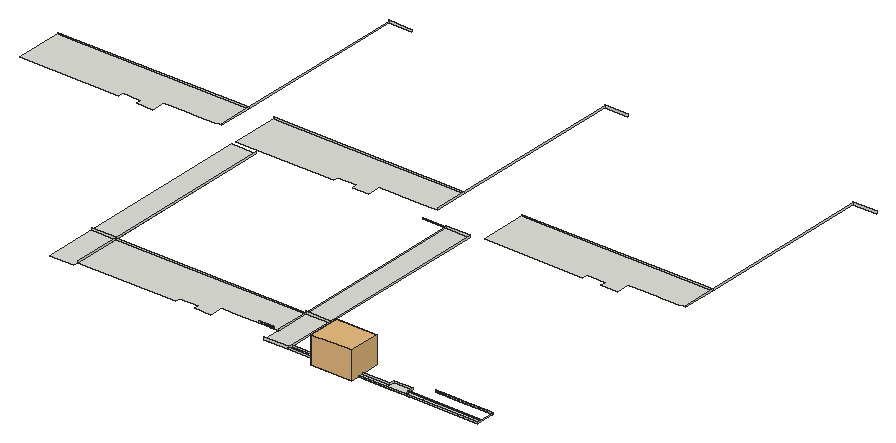
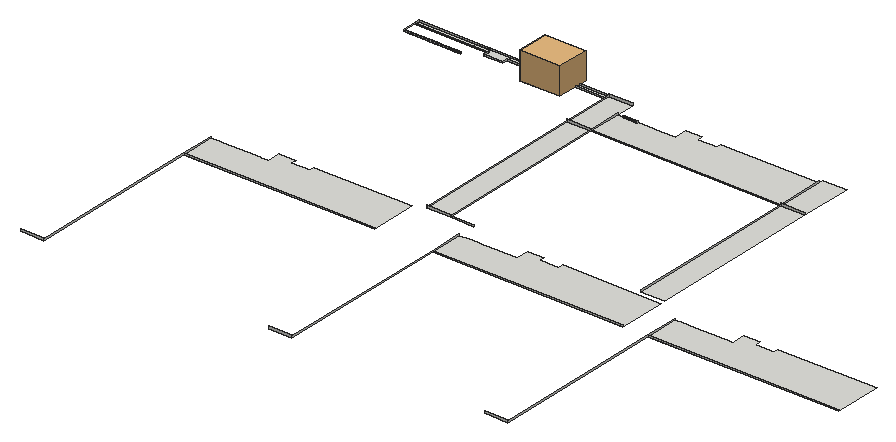
# SketchUp Ruby script. Lengths in inches.
U = 1.inch
M = Sketchup.active_model
def pt(a) = Geom::Point3d.new(a.map { |v| v * U })
def face(e, loops, mat)
  f = e.add_face(loops[0].map { |a| pt(a) })
  loops[1..].each { |l| e.add_face(l.map { |a| pt(a) }).erase! }
  f.material = f.back_material = mat if mat
  f
end
# faces: each face lists its corners as indices into pts; further lists are holes
def faces(e, pts, list, mat = nil) = list.each { |f| face(e, (f[0].is_a?(Array) ? f : [f]).map { |l| l.map { |i| pts[i] } }, mat) }
# xy, xz, yz: faces in a plane at the given z, y or x. An outline is a flat list of corners, or four numbers for a rectangle; further outlines are holes
def ring(l) = l.size == 4 ? [[l[0], l[1]], [l[2], l[1]], [l[2], l[3]], [l[0], l[3]]] : l.each_slice(2).to_a
def flat(e, list, mat, &to3) = list.each { |f| face(e, (f[0].is_a?(Array) ? f : [f]).map { |l| ring(l).map { |u, v| to3.(u, v) } }, mat) }
def xy(e, z, list, mat = nil) = flat(e, list, mat) { |x, y| [x, y, z] }
def xz(e, y, list, mat = nil) = flat(e, list, mat) { |x, z| [x, y, z] }
def yz(e, x, list, mat = nil) = flat(e, list, mat) { |y, z| [x, y, z] }
def lines(e, pts, list) = list.each { |a, b| e.add_line(pt(pts[a]), pt(pts[b])) }
# prism: a flat outline (further loops are holes) pulled along v
def prism(e, loops, v, mat = nil)
  f = face(e, loops, mat); d = Geom::Vector3d.new(v.map { |x| x * U })
  f.pushpull(f.normal.samedirection?(d) ? d.length : -d.length)
end
def box(e, o, s, mat = nil) = prism(e, [[o, [o[0] + s[0], o[1], o[2]], [o[0] + s[0], o[1] + s[1], o[2]], [o[0], o[1] + s[1], o[2]]]], [0, 0, s[2]], mat)
def at(x, y, z, deg = 0) = Geom::Transformation.translation(pt([x, y, z])) * Geom::Transformation.rotation(ORIGIN, Z_AXIS, deg.degrees)
def axes(o, x, y, z) = Geom::Transformation.new([*x, 0, *y, 0, *z, 0, *pt(o).to_a, 1])
def part(name) = M.definitions.add(name)
# library, detail: a bought-in or finely detailed component or shape, given as its bounding box
def library(name, o, s) = part(name).tap { |d| box(d.entities, o, s) }
def detail(e, o, s) = box(e.add_group.entities, o, s)
def put(e, d, t, mat = nil) = e.add_instance(d, t).tap { |i| i.material = mat if mat }
def group(e, t, mat = nil) = e.add_group.tap { |g| g.transformation = t; g.material = mat if mat }.entities
root = M.entities
c1 = library("Sem+nome (1)",[20.77,3.52,-2.22],[96.42,122.82,82.56])
xy(root,-12.3125,[[1063.02,147.25,1134.71,305.58],[1713.52,147.25,1785.21,305.58],[1785.21,147.25,1886.4,162.52],[1950.69,147.25,1952.69,147.38,1954.64,147.77,1956.53,148.41,1958.33,149.3,1959.99,150.4,1961.49,151.72,1962.8,153.22,1963.91,154.88,1964.8,156.67,1965.4375,158.57,1965.83,160.52,1965.96,162.52,2083.4,162.52,2083.4,147.25],[2083.4,147.25,2083.4,178.0625,2140.42,178.0625,2140.42,162.33,2140.55,160.36,2140.93,158.43,2141.57,156.56,2142.4375,154.79,2143.53,153.15,2144.84,151.67,2146.32,150.37,2147.96,149.27,2149.73,148.4,2151.6,147.76,2153.53,147.38,2155.5,147.25],
  [2155.5,147.25,2153.53,147.38,2151.6,147.76,2149.73,148.4,2147.96,149.27,2146.32,150.37,2144.84,151.67,2143.53,153.15,2142.4375,154.79,2141.57,156.56,2140.93,158.43,2140.55,160.36,2140.42,162.33,2189.5,162.33,2189.5,147.25],[2189.5,147.25,2364.02,162.33],[1489.92,162.33,1489.92,178.0625,1432.9,178.0625,1432.9,162.52,1134.71,162.52,1134.71,305.58,1713.52,305.58,1713.52,203.875,1697.375,203.875,1697.375,204.875,1696.625,204.875,1696.625,203.875,1693.375,203.875,1693.375,204.875,1692.625,204.875,1692.625,203.875,1689.375,203.875,1689.375,204.875,1688.625,204.875,1688.625,203.875,1685.375,203.875,1685.375,204.875,1684.625,204.875,1684.625,203.875,1681.375,203.875,1681.375,204.875,1680.625,204.875,1680.625,203.875,1677.375,203.875,1677.375,204.875,1676.625,204.875,1676.625,203.875,1673.375,203.875,1673.375,204.875,1672.625,204.875,1672.625,203.875,1669.375,203.875,1669.375,204.875,1668.625,204.875,1668.625,203.875,1665.375,203.875,1665.375,204.875,1664.625,204.875,1664.625,203.875,1661.375,203.875,1661.375,204.875,1660.625,204.875,1660.625,203.875,1657.375,203.875,1657.375,204.875,1656.625,204.875,1656.625,203.875,1653.375,203.875,1653.375,204.875,1652.625,204.875,1652.625,203.875,1649.375,203.875,1649.375,204.875,1648.625,204.875,1648.625,203.875,1645.375,203.875,1645.375,204.875,1644.625,204.875,1644.625,203.875,1641.375,203.875,1641.375,204.875,1640.625,204.875,1640.625,203.875,1637.375,203.875,1637.375,204.875,1636.625,204.875,1636.625,203.875,1633.375,203.875,1633.375,204.875,1632.625,204.875,1632.625,203.875,1629.375,203.875,1629.375,204.875,1628.625,204.875,1628.625,203.875,1625.375,203.875,1625.375,204.875,1624.625,204.875,1624.625,203.875,1621.375,203.875,1621.375,204.875,1620.625,204.875,1620.625,203.875,1617.375,203.875,1617.375,204.875,1616.625,204.875,1616.625,203.875,1613.375,203.875,1613.375,204.875,1612.625,204.875,1612.625,203.875,1609.375,203.875,1609.375,204.875,1608.625,204.875,1608.625,203.875,1605.375,203.875,1605.375,204.875,1604.625,204.875,1604.625,203.875,1601.375,203.875,1601.375,204.875,1600.625,204.875,1600.625,203.875,1597.375,203.875,1597.375,204.875,1596.625,204.875,1596.625,203.875,1593.375,203.875,1593.375,204.875,1592.625,204.875,1592.625,203.875,1589.375,203.875,1589.375,204.875,1588.625,204.875,1588.625,203.875,1585.375,203.875,1585.375,204.875,1584.625,204.875,1584.625,203.875,1581.375,203.875,1581.375,204.875,1580.625,204.875,1580.625,203.875,1577.375,203.875,1577.375,204.875,1576.625,204.875,1576.625,203.875,1573.375,203.875,1573.375,204.875,1572.625,204.875,1572.625,203.875,1569.375,203.875,1569.375,204.875,1568.625,204.875,1568.625,203.875,1565.375,203.875,1565.375,204.875,1564.625,204.875,1564.625,203.875,1561.375,203.875,1561.375,204.875,1560.625,204.875,1560.625,203.875,1557.375,203.875,1557.375,204.875,1556.625,204.875,1556.625,203.875,1553.375,203.875,1553.375,204.875,1552.625,204.875,1552.625,203.875,1549.375,203.875,1549.375,204.875,1548.625,204.875,1548.625,203.875,1545.375,203.875,1545.375,204.875,1544.625,204.875,1544.625,203.875,1541.375,203.875,1541.375,204.875,1540.625,204.875,1540.625,203.875,1539,203.875,1539,162.33],[1063.02,305.58,1134.71,838.14],[1713.52,305.58,1785.21,838.14],
  [762.73,853.22,762.73,868.96,705.71,868.96,705.71,853.41,407.52,853.41,407.52,996.48,986.33,996.48,986.33,894.77,970.1875,894.77,970.1875,895.77,969.4375,895.77,969.4375,894.77,966.1875,894.77,966.1875,895.77,965.4375,895.77,965.4375,894.77,962.1875,894.77,962.1875,895.77,961.4375,895.77,961.4375,894.77,958.1875,894.77,958.1875,895.77,957.4375,895.77,957.4375,894.77,954.1875,894.77,954.1875,895.77,953.4375,895.77,953.4375,894.77,950.1875,894.77,950.1875,895.77,949.4375,895.77,949.4375,894.77,946.1875,894.77,946.1875,895.77,945.4375,895.77,945.4375,894.77,942.1875,894.77,942.1875,895.77,941.4375,895.77,941.4375,894.77,938.1875,894.77,938.1875,895.77,937.4375,895.77,937.4375,894.77,934.1875,894.77,934.1875,895.77,933.4375,895.77,933.4375,894.77,930.1875,894.77,930.1875,895.77,929.4375,895.77,929.4375,894.77,926.1875,894.77,926.1875,895.77,925.4375,895.77,925.4375,894.77,922.1875,894.77,922.1875,895.77,921.4375,895.77,921.4375,894.77,918.1875,894.77,918.1875,895.77,917.4375,895.77,917.4375,894.77,914.1875,894.77,914.1875,895.77,913.4375,895.77,913.4375,894.77,910.1875,894.77,910.1875,895.77,909.4375,895.77,909.4375,894.77,906.1875,894.77,906.1875,895.77,905.4375,895.77,905.4375,894.77,902.1875,894.77,902.1875,895.77,901.4375,895.77,901.4375,894.77,898.1875,894.77,898.1875,895.77,897.4375,895.77,897.4375,894.77,894.1875,894.77,894.1875,895.77,893.4375,895.77,893.4375,894.77,890.1875,894.77,890.1875,895.77,889.4375,895.77,889.4375,894.77,886.1875,894.77,886.1875,895.77,885.4375,895.77,885.4375,894.77,882.1875,894.77,882.1875,895.77,881.4375,895.77,881.4375,894.77,878.1875,894.77,878.1875,895.77,877.4375,895.77,877.4375,894.77,874.1875,894.77,874.1875,895.77,873.4375,895.77,873.4375,894.77,870.1875,894.77,870.1875,895.77,869.4375,895.77,869.4375,894.77,866.1875,894.77,866.1875,895.77,865.4375,895.77,865.4375,894.77,862.1875,894.77,862.1875,895.77,861.4375,895.77,861.4375,894.77,858.1875,894.77,858.1875,895.77,857.4375,895.77,857.4375,894.77,854.1875,894.77,854.1875,895.77,853.4375,895.77,853.4375,894.77,850.1875,894.77,850.1875,895.77,849.4375,895.77,849.4375,894.77,846.1875,894.77,846.1875,895.77,845.4375,895.77,845.4375,894.77,842.1875,894.77,842.1875,895.77,841.4375,895.77,841.4375,894.77,838.1875,894.77,838.1875,895.77,837.4375,895.77,837.4375,894.77,834.1875,894.77,834.1875,895.77,833.4375,895.77,833.4375,894.77,830.1875,894.77,830.1875,895.77,829.4375,895.77,829.4375,894.77,826.1875,894.77,826.1875,895.77,825.4375,895.77,825.4375,894.77,822.1875,894.77,822.1875,895.77,821.4375,895.77,821.4375,894.77,818.1875,894.77,818.1875,895.77,817.4375,895.77,817.4375,894.77,814.1875,894.77,814.1875,895.77,813.4375,895.77,813.4375,894.77,811.8125,894.77,811.8125,853.22],[1418.23,853.22,1418.23,868.96,1361.21,868.96,1361.21,853.41,1063.02,853.41,1063.02,996.48,1641.83,996.48,1641.83,894.77,1625.6875,894.77,1625.6875,895.77,1624.9375,895.77,1624.9375,894.77,1621.6875,894.77,1621.6875,895.77,1620.9375,895.77,1620.9375,894.77,1617.6875,894.77,1617.6875,895.77,1616.9375,895.77,1616.9375,894.77,1613.6875,894.77,1613.6875,895.77,1612.9375,895.77,1612.9375,894.77,1609.6875,894.77,1609.6875,895.77,1608.9375,895.77,1608.9375,894.77,1605.6875,894.77,1605.6875,895.77,1604.9375,895.77,1604.9375,894.77,1601.6875,894.77,1601.6875,895.77,1600.9375,895.77,1600.9375,894.77,1597.6875,894.77,1597.6875,895.77,1596.9375,895.77,1596.9375,894.77,1593.6875,894.77,1593.6875,895.77,1592.9375,895.77,1592.9375,894.77,1589.6875,894.77,1589.6875,895.77,1588.9375,895.77,1588.9375,894.77,1585.6875,894.77,1585.6875,895.77,1584.9375,895.77,1584.9375,894.77,1581.6875,894.77,1581.6875,895.77,1580.9375,895.77,1580.9375,894.77,1577.6875,894.77,1577.6875,895.77,1576.9375,895.77,1576.9375,894.77,1573.6875,894.77,1573.6875,895.77,1572.9375,895.77,1572.9375,894.77,1569.6875,894.77,1569.6875,895.77,1568.9375,895.77,1568.9375,894.77,1565.6875,894.77,1565.6875,895.77,1564.9375,895.77,1564.9375,894.77,1561.6875,894.77,1561.6875,895.77,1560.9375,895.77,1560.9375,894.77,1557.6875,894.77,1557.6875,895.77,1556.9375,895.77,1556.9375,894.77,1553.6875,894.77,1553.6875,895.77,1552.9375,895.77,1552.9375,894.77,1549.6875,894.77,1549.6875,895.77,1548.9375,895.77,1548.9375,894.77,1545.6875,894.77,1545.6875,895.77,1544.9375,895.77,1544.9375,894.77,1541.6875,894.77,1541.6875,895.77,1540.9375,895.77,1540.9375,894.77,1537.6875,894.77,1537.6875,895.77,1536.9375,895.77,1536.9375,894.77,1533.6875,894.77,1533.6875,895.77,1532.9375,895.77,1532.9375,894.77,1529.6875,894.77,1529.6875,895.77,1528.9375,895.77,1528.9375,894.77,1525.6875,894.77,1525.6875,895.77,1524.9375,895.77,1524.9375,894.77,1521.6875,894.77,1521.6875,895.77,1520.9375,895.77,1520.9375,894.77,1517.6875,894.77,1517.6875,895.77,1516.9375,895.77,1516.9375,894.77,1513.6875,894.77,1513.6875,895.77,1512.9375,895.77,1512.9375,894.77,1509.6875,894.77,1509.6875,895.77,1508.9375,895.77,1508.9375,894.77,1505.6875,894.77,1505.6875,895.77,1504.9375,895.77,1504.9375,894.77,1501.6875,894.77,1501.6875,895.77,1500.9375,895.77,1500.9375,894.77,1497.6875,894.77,1497.6875,895.77,1496.9375,895.77,1496.9375,894.77,1493.6875,894.77,1493.6875,895.77,1492.9375,895.77,1492.9375,894.77,1489.6875,894.77,1489.6875,895.77,1488.9375,895.77,1488.9375,894.77,1485.6875,894.77,1485.6875,895.77,1484.9375,895.77,1484.9375,894.77,1481.6875,894.77,1481.6875,895.77,1480.9375,895.77,1480.9375,894.77,1477.6875,894.77,1477.6875,895.77,1476.9375,895.77,1476.9375,894.77,1473.6875,894.77,1473.6875,895.77,1472.9375,895.77,1472.9375,894.77,1469.6875,894.77,1469.6875,895.77,1468.9375,895.77,1468.9375,894.77,1467.3125,894.77,1467.3125,853.22],[2172.86,853.22,2172.86,868.96,2115.83,868.96,2115.83,853.41,1817.65,853.41,1817.65,996.48,2396.46,996.48,2396.46,894.77,2380.3125,894.77,2380.3125,895.77,2379.5625,895.77,2379.5625,894.77,2376.3125,894.77,2376.3125,895.77,2375.5625,895.77,2375.5625,894.77,2372.3125,894.77,2372.3125,895.77,2371.5625,895.77,2371.5625,894.77,2368.3125,894.77,2368.3125,895.77,2367.5625,895.77,2367.5625,894.77,2364.3125,894.77,2364.3125,895.77,2363.5625,895.77,2363.5625,894.77,2360.3125,894.77,2360.3125,895.77,2359.5625,895.77,2359.5625,894.77,2356.3125,894.77,2356.3125,895.77,2355.5625,895.77,2355.5625,894.77,2352.3125,894.77,2352.3125,895.77,2351.5625,895.77,2351.5625,894.77,2348.3125,894.77,2348.3125,895.77,2347.5625,895.77,2347.5625,894.77,2344.3125,894.77,2344.3125,895.77,2343.5625,895.77,2343.5625,894.77,2340.3125,894.77,2340.3125,895.77,2339.5625,895.77,2339.5625,894.77,2336.3125,894.77,2336.3125,895.77,2335.5625,895.77,2335.5625,894.77,2332.3125,894.77,2332.3125,895.77,2331.5625,895.77,2331.5625,894.77,2328.3125,894.77,2328.3125,895.77,2327.5625,895.77,2327.5625,894.77,2324.3125,894.77,2324.3125,895.77,2323.5625,895.77,2323.5625,894.77,2320.3125,894.77,2320.3125,895.77,2319.5625,895.77,2319.5625,894.77,2316.3125,894.77,2316.3125,895.77,2315.5625,895.77,2315.5625,894.77,2312.3125,894.77,2312.3125,895.77,2311.5625,895.77,2311.5625,894.77,2308.3125,894.77,2308.3125,895.77,2307.5625,895.77,2307.5625,894.77,2304.3125,894.77,2304.3125,895.77,2303.5625,895.77,2303.5625,894.77,2300.3125,894.77,2300.3125,895.77,2299.5625,895.77,2299.5625,894.77,2296.3125,894.77,2296.3125,895.77,2295.5625,895.77,2295.5625,894.77,2292.3125,894.77,2292.3125,895.77,2291.5625,895.77,2291.5625,894.77,2288.3125,894.77,2288.3125,895.77,2287.5625,895.77,2287.5625,894.77,2284.3125,894.77,2284.3125,895.77,2283.5625,895.77,2283.5625,894.77,2280.3125,894.77,2280.3125,895.77,2279.5625,895.77,2279.5625,894.77,2276.3125,894.77,2276.3125,895.77,2275.5625,895.77,2275.5625,894.77,2272.3125,894.77,2272.3125,895.77,2271.5625,895.77,2271.5625,894.77,2268.3125,894.77,2268.3125,895.77,2267.5625,895.77,2267.5625,894.77,2264.3125,894.77,2264.3125,895.77,2263.5625,895.77,2263.5625,894.77,2260.3125,894.77,2260.3125,895.77,2259.5625,895.77,2259.5625,894.77,2256.3125,894.77,2256.3125,895.77,2255.5625,895.77,2255.5625,894.77,2252.3125,894.77,2252.3125,895.77,2251.5625,895.77,2251.5625,894.77,2248.3125,894.77,2248.3125,895.77,2247.5625,895.77,2247.5625,894.77,2244.3125,894.77,2244.3125,895.77,2243.5625,895.77,2243.5625,894.77,2240.3125,894.77,2240.3125,895.77,2239.5625,895.77,2239.5625,894.77,2236.3125,894.77,2236.3125,895.77,2235.5625,895.77,2235.5625,894.77,2232.3125,894.77,2232.3125,895.77,2231.5625,895.77,2231.5625,894.77,2228.3125,894.77,2228.3125,895.77,2227.5625,895.77,2227.5625,894.77,2224.3125,894.77,2224.3125,895.77,2223.5625,895.77,2223.5625,894.77,2221.9375,894.77,2221.9375,853.22]])
xz(root,147.25,[[1713.52,-12.3125,1785.21,-4.67],[1785.21,-12.3125,1886.4,-8],[1886.4,-12.3125,1950.69,-8],[1950.69,-12.3125,2364.02,-8]])
xz(root,162.33,[[2140.42,-12.3125,2364.02,-8]])
xz(root,162.52,[[1785.21,-12.3125,1886.4,-8],[1886.4,-12.3125,1965.96,-8],[1965.96,-12.3125,2083.4,-8]])
xz(root,178.0625,[[2083.4,-12.3125,2140.42,-8]])
xz(root,203.875,[[2189.5,-12.3125,2191.125,-8],[2191.875,-12.3125,2195.125,-8],[2195.875,-12.3125,2199.125,-8],[2199.875,-12.3125,2203.125,-8],[2203.875,-12.3125,2207.125,-8],
  [2207.875,-12.3125,2211.125,-8],[2211.875,-12.3125,2215.125,-8],[2215.875,-12.3125,2219.125,-8],[2219.875,-12.3125,2223.125,-8],[2223.875,-12.3125,2227.125,-8],
  [2227.875,-12.3125,2231.125,-8],[2231.875,-12.3125,2235.125,-8],[2235.875,-12.3125,2239.125,-8],[2239.875,-12.3125,2243.125,-8],[2243.875,-12.3125,2247.125,-8],
  [2247.875,-12.3125,2251.125,-8],[2251.875,-12.3125,2255.125,-8],[2255.875,-12.3125,2259.125,-8],[2259.875,-12.3125,2263.125,-8],[2263.875,-12.3125,2267.125,-8],
  [2267.875,-12.3125,2271.125,-8],[2271.875,-12.3125,2275.125,-8],[2275.875,-12.3125,2279.125,-8],[2279.875,-12.3125,2283.125,-8],[2283.875,-12.3125,2287.125,-8],
  [2287.875,-12.3125,2291.125,-8],[2291.875,-12.3125,2295.125,-8],[2295.875,-12.3125,2299.125,-8],[2299.875,-12.3125,2303.125,-8],[2303.875,-12.3125,2307.125,-8],
  [2307.875,-12.3125,2311.125,-8],[2311.875,-12.3125,2315.125,-8],[2315.875,-12.3125,2319.125,-8],[2319.875,-12.3125,2323.125,-8],[2323.875,-12.3125,2327.125,-8],
  [2327.875,-12.3125,2331.125,-8],[2331.875,-12.3125,2335.125,-8],[2335.875,-12.3125,2339.125,-8],[2339.875,-12.3125,2343.125,-8],[2343.875,-12.3125,2347.125,-8],
  [2347.875,-12.3125,2351.125,-8],[2351.125,-12.3125,2364.02,-8]])
xz(root,204.875,[[1656.625,-12.3125,1657.375,-8],[1660.625,-12.3125,1661.375,-8],[1664.625,-12.3125,1665.375,-8],[1668.625,-12.3125,1669.375,-8],[1672.625,-12.3125,1673.375,-8],
  [1676.625,-12.3125,1677.375,-8],[1680.625,-12.3125,1681.375,-8],[1684.625,-12.3125,1685.375,-8],[1688.625,-12.3125,1689.375,-8],[1692.625,-12.3125,1693.375,-8],
  [1696.625,-12.3125,1697.375,-8],[2199.125,-12.3125,2199.875,-8],[2203.125,-12.3125,2203.875,-8],[2207.125,-12.3125,2207.875,-8],[2211.125,-12.3125,2211.875,-8],
  [2219.125,-12.3125,2219.875,-8]])
xz(root,305.58,[[1063.02,-12.3125,1134.71,-4.67],[1134.71,-12.3125,1713.52,-8],[1713.52,-12.3125,1785.21,-4.67]])
xz(root,838.14,[[1641.83,-12.3125,1713.52,-8],[1713.52,-12.3125,1785.21,-4.67]])
xz(root,996.48,[[407.52,-12.3125,986.33,-8],[1063.02,-12.3125,1641.83,-8],[1817.65,-12.3125,2396.46,-8]])
xz(root,1529.04,[[986.33,-12.3125,1058.02,-4.67],[1641.83,-12.3125,1713.52,-4.67],[2396.46,-12.3125,2468.15,-4.67]])
yz(root,986.33,[[894.77,-12.3125,996.48,-8],[996.48,-12.3125,1529.04,-8]])
yz(root,1134.71,[[162.52,-12.3125,305.58,-8],[305.58,-12.3125,838.14,-8]])
yz(root,1641.83,[[894.77,-12.3125,996.48,-8],[996.48,-12.3125,1529.04,-8]])
yz(root,1653.375,[[203.875,-12.3125,204.875,-8]])
yz(root,1656.625,[[203.875,-12.3125,204.875,-8]])
yz(root,1657.375,[[203.875,-12.3125,204.875,-8]])
yz(root,1660.625,[[203.875,-12.3125,204.875,-8]])
yz(root,1661.375,[[203.875,-12.3125,204.875,-8]])
yz(root,1664.625,[[203.875,-12.3125,204.875,-8]])
yz(root,1665.375,[[203.875,-12.3125,204.875,-8]])
yz(root,1668.625,[[203.875,-12.3125,204.875,-8]])
yz(root,1669.375,[[203.875,-12.3125,204.875,-8]])
yz(root,1672.625,[[203.875,-12.3125,204.875,-8]])
yz(root,1673.375,[[203.875,-12.3125,204.875,-8]])
yz(root,1676.625,[[203.875,-12.3125,204.875,-8]])
yz(root,1677.375,[[203.875,-12.3125,204.875,-8]])
yz(root,1680.625,[[203.875,-12.3125,204.875,-8]])
yz(root,1681.375,[[203.875,-12.3125,204.875,-8]])
yz(root,1684.625,[[203.875,-12.3125,204.875,-8]])
yz(root,1685.375,[[203.875,-12.3125,204.875,-8]])
yz(root,1688.625,[[203.875,-12.3125,204.875,-8]])
yz(root,1689.375,[[203.875,-12.3125,204.875,-8]])
yz(root,1692.625,[[203.875,-12.3125,204.875,-8]])
yz(root,1693.375,[[203.875,-12.3125,204.875,-8]])
yz(root,1696.625,[[203.875,-12.3125,204.875,-8]])
yz(root,1697.375,[[203.875,-12.3125,204.875,-8]])
yz(root,1713.52,[[203.875,-12.3125,305.58,-8],[305.58,-12.3125,838.14,-8]])
yz(root,1785.21,[[147.25,-12.3125,162.52,-8],[162.52,-12.3125,305.58,-8],[305.58,-12.3125,838.14,-8]])
yz(root,1886.4,[[147.25,-12.3125,162.52,-8]])
yz(root,2083.4,[[162.52,-12.3125,178.0625,-8]])
yz(root,2140.42,[[162.33,-12.3125,178.0625,-8]])
yz(root,2195.875,[[203.875,-12.3125,204.875,-8]])
yz(root,2199.125,[[203.875,-12.3125,204.875,-8]])
yz(root,2199.875,[[203.875,-12.3125,204.875,-8]])
yz(root,2203.125,[[203.875,-12.3125,204.875,-8]])
yz(root,2203.875,[[203.875,-12.3125,204.875,-8]])
yz(root,2207.125,[[203.875,-12.3125,204.875,-8]])
yz(root,2211.875,[[203.875,-12.3125,204.875,-8]])
yz(root,2215.125,[[203.875,-12.3125,204.875,-8]])
yz(root,2215.875,[[203.875,-12.3125,204.875,-8]])
yz(root,2219.125,[[203.875,-12.3125,204.875,-8]])
yz(root,2219.875,[[203.875,-12.3125,204.875,-8]])
yz(root,2364.02,[[147.25,-12.3125,162.33,-8],[162.33,-12.3125,198.625,-8],[198.625,-12.3125,203.875,-8]])
yz(root,2396.46,[[894.77,-12.3125,996.48,-8],[996.48,-12.3125,1529.04,-8]])
p = [[1952.69,147.38,-8],[1950.69,147.25,-8],[1950.69,147.25,-12.3125],[1952.69,147.38,-12.3125],[1954.64,147.77,-8],[1954.64,147.77,-12.3125],
  [2153.53,147.38,-8],[2151.6,147.76,-8],[2151.6,147.76,-12.3125],[2153.53,147.38,-12.3125],[1956.53,148.41,-8],[1956.53,148.41,-12.3125],
  [2149.73,148.4,-8],[2149.73,148.4,-12.3125],[1958.33,149.3,-8],[1958.33,149.3,-12.3125],[2147.96,149.27,-8],[2147.96,149.27,-12.3125],
  [1959.99,150.4,-8],[1959.99,150.4,-12.3125],[2146.32,150.37,-8],[2146.32,150.37,-12.3125],[1961.49,151.72,-8],[1961.49,151.72,-12.3125],
  [2144.84,151.67,-8],[2144.84,151.67,-12.3125],[1962.8,153.22,-8],[1962.8,153.22,-12.3125],[2143.53,153.15,-8],[2143.53,153.15,-12.3125],
  [1963.91,154.88,-8],[1963.91,154.88,-12.3125],[2142.4375,154.79,-8],[2142.4375,154.79,-12.3125],[2141.57,156.56,-8],[2141.57,156.56,-12.3125],
  [1964.8,156.67,-8],[1964.8,156.67,-12.3125],[2140.93,158.43,-8],[2140.93,158.43,-12.3125],[1965.4375,158.57,-8],[1965.4375,158.57,-12.3125],
  [2140.55,160.36,-8],[2140.55,160.36,-12.3125],[1965.83,160.52,-8],[1965.83,160.52,-12.3125],[2140.42,162.33,-8],[2140.42,162.33,-12.3125],
  [1965.96,162.52,-8],[1965.96,162.52,-12.3125],[1058.02,838.14,-12.3125],[1058.02,838.14,-8]]
faces(root,p,[[0,1,2,3],[4,0,3,5],[6,7,8,9],[10,4,5,11],[7,12,13,8],[14,10,11,15],[12,16,17,13],[18,14,15,19],
  [16,20,21,17],[22,18,19,23],[20,24,25,21],[26,22,23,27],[24,28,29,25],[30,26,27,31],[28,32,33,29],[32,34,35,33],
  [36,30,31,37],[34,38,39,35],[40,36,37,41],[38,42,43,39],[44,40,41,45],[42,46,47,43],[48,44,45,49]])
lines(root,p,[[50,51]])
put(root,c1,at(1872.48,239.07,-10.09,-90))
